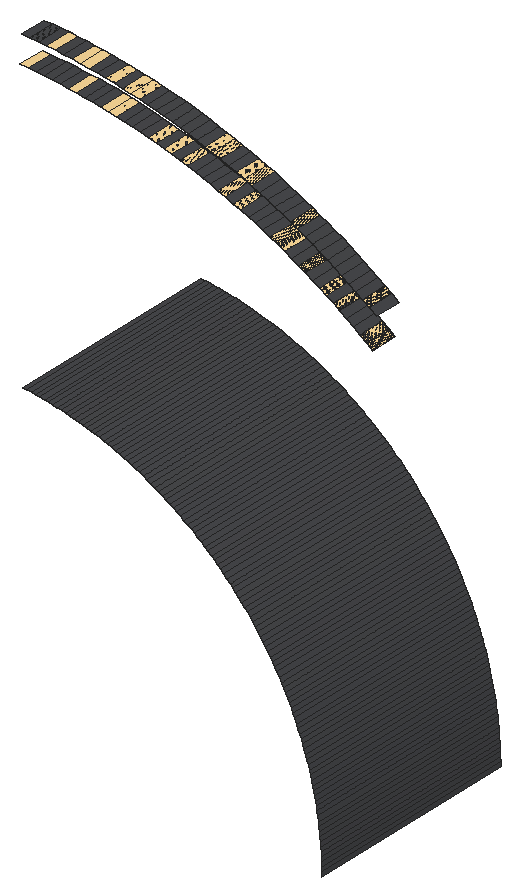
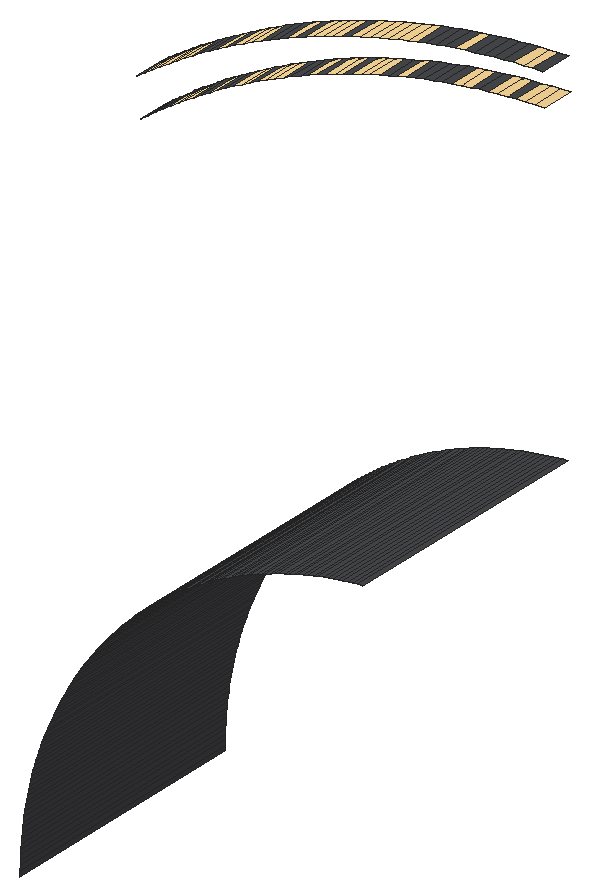
# SketchUp Ruby script. Lengths in inches.
U = 1.inch
M = Sketchup.active_model
def pt(a) = Geom::Point3d.new(a.map { |v| v * U })
def face(e, loops, mat)
  f = e.add_face(loops[0].map { |a| pt(a) })
  loops[1..].each { |l| e.add_face(l.map { |a| pt(a) }).erase! }
  f.material = f.back_material = mat if mat
  f
end
# faces: each face lists its corners as indices into pts; further lists are holes
def faces(e, pts, list, mat = nil) = list.each { |f| face(e, (f[0].is_a?(Array) ? f : [f]).map { |l| l.map { |i| pts[i] } }, mat) }
# xy, xz, yz: faces in a plane at the given z, y or x. An outline is a flat list of corners, or four numbers for a rectangle; further outlines are holes
def ring(l) = l.size == 4 ? [[l[0], l[1]], [l[2], l[1]], [l[2], l[3]], [l[0], l[3]]] : l.each_slice(2).to_a
def flat(e, list, mat, &to3) = list.each { |f| face(e, (f[0].is_a?(Array) ? f : [f]).map { |l| ring(l).map { |u, v| to3.(u, v) } }, mat) }
def xy(e, z, list, mat = nil) = flat(e, list, mat) { |x, y| [x, y, z] }
def xz(e, y, list, mat = nil) = flat(e, list, mat) { |x, z| [x, y, z] }
def yz(e, x, list, mat = nil) = flat(e, list, mat) { |y, z| [x, y, z] }
def lines(e, pts, list) = list.each { |a, b| e.add_line(pt(pts[a]), pt(pts[b])) }
# prism: a flat outline (further loops are holes) pulled along v
def prism(e, loops, v, mat = nil)
  f = face(e, loops, mat); d = Geom::Vector3d.new(v.map { |x| x * U })
  f.pushpull(f.normal.samedirection?(d) ? d.length : -d.length)
end
def box(e, o, s, mat = nil) = prism(e, [[o, [o[0] + s[0], o[1], o[2]], [o[0] + s[0], o[1] + s[1], o[2]], [o[0], o[1] + s[1], o[2]]]], [0, 0, s[2]], mat)
def at(x, y, z, deg = 0) = Geom::Transformation.translation(pt([x, y, z])) * Geom::Transformation.rotation(ORIGIN, Z_AXIS, deg.degrees)
def axes(o, x, y, z) = Geom::Transformation.new([*x, 0, *y, 0, *z, 0, *pt(o).to_a, 1])
def part(name) = M.definitions.add(name)
# library, detail: a bought-in or finely detailed component or shape, given as its bounding box
def library(name, o, s) = part(name).tap { |d| box(d.entities, o, s) }
def detail(e, o, s) = box(e.add_group.entities, o, s)
def put(e, d, t, mat = nil) = e.add_instance(d, t).tap { |i| i.material = mat if mat }
def group(e, t, mat = nil) = e.add_group.tap { |g| g.transformation = t; g.material = mat if mat }.entities
root = M.entities
M.materials.add("1432 AP 8245 TAR ROAD").color = [71, 72, 75]
M.materials.add("Outer Light").color = [251, 217, 152]
yz(root,410.99,[[95.37,411.26,107.37,411.5]],"1432 AP 8245 TAR ROAD")
yz(root,411,[[95.37,410.79,107.37,411.03]],"1432 AP 8245 TAR ROAD")
p = [[410.99,107.37,411.26],[411,107.37,411.03],[411,95.37,411.03],[410.99,95.37,411.26],[410.98,107.37,411.73],[410.99,107.37,411.5],
  [410.99,95.37,411.5],[410.98,95.37,411.73],[410.96,107.37,411.97],[410.96,95.37,411.97],[410.94,107.37,412.2],[410.94,95.37,412.2],
  [410.92,107.37,412.4375],[410.92,95.37,412.4375],[410.9,107.37,412.67],[410.9,95.37,412.67],[410.875,107.37,412.91],[410.875,95.37,412.91],
  [410.85,107.37,413.14],[410.85,95.37,413.14],[410.8125,107.37,413.375],[410.8125,95.37,413.375],[410.78,107.37,413.61],[410.78,95.37,413.61],
  [410.74,107.37,413.84],[410.74,95.37,413.84],[410.7,107.37,414.07],[410.7,95.37,414.07],[410.65,107.37,414.3],[410.65,95.37,414.3],
  [410.61,107.37,414.53],[410.61,95.37,414.53],[410.56,107.37,414.76],[410.56,95.37,414.76],[410.5,107.37,414.99],[410.5,95.37,414.99],
  [410.45,107.37,415.22],[410.45,95.37,415.22],[410.39,107.37,415.45],[410.39,95.37,415.45],[410.32,107.37,415.68],[410.32,95.37,415.68],
  [410.26,107.37,415.9],[410.26,95.37,415.9],[410.19,107.37,416.13],[410.19,95.37,416.13],[410.12,107.37,416.35],[410.12,95.37,416.35],
  [410.04,107.37,416.58],[410.04,95.37,416.58],[409.97,107.37,416.8],[409.97,95.37,416.8],[409.89,107.37,417.02],[409.89,95.37,417.02],
  [409.8,107.37,417.24],[409.8,95.37,417.24],[409.72,107.37,417.46],[409.72,95.37,417.46],[409.63,107.37,417.68],[409.63,95.37,417.68],
  [409.54,107.37,417.9],[409.54,95.37,417.9],[409.44,107.37,418.11],[409.44,95.37,418.11],[409.35,107.37,418.33],[409.35,95.37,418.33],
  [409.25,107.37,418.54],[409.25,95.37,418.54],[409.14,107.37,418.75],[409.14,95.37,418.75],[409.04,107.37,418.96],[409.04,95.37,418.96],
  [408.93,107.37,419.17],[408.93,95.37,419.17],[408.82,107.37,419.38],[408.82,95.37,419.38],[408.7,107.37,419.59],[408.7,95.37,419.59],
  [408.59,107.37,419.79],[408.59,95.37,419.79],[408.47,107.37,420],[408.47,95.37,420],[408.35,107.37,420.2],[408.35,95.37,420.2],
  [408.22,107.37,420.4],[408.22,95.37,420.4],[408.1,107.37,420.6],[408.1,95.37,420.6],[407.97,107.37,420.79],[407.97,95.37,420.79],
  [407.83,107.37,420.99],[407.83,95.37,420.99],[407.7,107.37,421.18],[407.7,95.37,421.18],[407.5625,107.37,421.37],[407.5625,95.37,421.37],
  [407.42,107.37,421.5625],[407.42,95.37,421.5625],[407.28,107.37,421.75],[407.28,95.37,421.75],[407.14,107.37,421.9375],[407.14,95.37,421.9375],
  [406.99,107.37,422.12],[406.99,95.37,422.12],[406.84,107.37,422.3],[406.84,95.37,422.3],[406.6875,107.37,422.48],[406.6875,95.37,422.48],
  [406.53,107.37,422.66],[406.53,95.37,422.66],[406.375,107.37,422.84],[406.375,95.37,422.84],[406.22,107.37,423.01],[406.22,95.37,423.01],
  [406.06,107.37,423.18],[406.06,95.37,423.18],[405.89,107.37,423.35],[405.89,95.37,423.35],[405.73,107.37,423.52],[405.73,95.37,423.52],
  [405.56,107.37,423.69],[405.56,95.37,423.69],[405.39,107.37,423.85],[405.39,95.37,423.85],[405.22,107.37,424.01],[405.22,95.37,424.01],
  [405.04,107.37,424.17],[405.04,95.37,424.17],[404.87,107.37,424.33],[404.87,95.37,424.33],[404.69,107.37,424.48],[404.69,95.37,424.48],
  [404.51,107.37,424.63],[404.51,95.37,424.63],[404.33,107.37,424.78],[404.33,95.37,424.78],[404.14,107.37,424.93],[404.14,95.37,424.93],
  [403.96,107.37,425.07],[403.96,95.37,425.07],[403.77,107.37,425.21],[403.77,95.37,425.21],[403.58,107.37,425.35],[403.58,95.37,425.35],
  [403.39,107.37,425.49],[403.39,95.37,425.49],[403.2,107.37,425.625],[403.2,95.37,425.625],[403,107.37,425.76],[403,95.37,425.76],
  [402.8,107.37,425.89],[402.8,95.37,425.89],[402.61,107.37,426.02],[402.61,95.37,426.02],[402.4,107.37,426.14],[402.4,95.37,426.14],
  [402.2,107.37,426.26],[402.2,95.37,426.26],[402,107.37,426.38],[402,95.37,426.38],[401.8,107.37,426.5],[401.8,95.37,426.5],
  [401.59,107.37,426.61],[401.59,95.37,426.61],[401.38,107.37,426.72],[401.38,95.37,426.72],[401.17,107.37,426.83],[401.17,95.37,426.83],
  [400.96,107.37,426.9375],[400.96,95.37,426.9375],[400.75,107.37,427.04],[400.75,95.37,427.04],[400.54,107.37,427.14],[400.54,95.37,427.14],
  [400.32,107.37,427.24],[400.32,95.37,427.24],[400.11,107.37,427.33],[400.11,95.37,427.33],[399.89,107.37,427.42],[399.89,95.37,427.42],
  [399.67,107.37,427.51],[399.67,95.37,427.51],[399.45,107.37,427.6],[399.45,95.37,427.6],[399.23,107.37,427.68],[399.23,95.37,427.68],
  [399.01,107.37,427.76],[399.01,95.37,427.76],[398.5625,107.37,427.91],[398.79,107.37,427.84],[398.79,95.37,427.84],[398.5625,95.37,427.91],
  [398.34,107.37,427.98],[398.34,95.37,427.98],[398.11,107.37,428.05],[398.11,95.37,428.05],[397.66,107.37,428.18],[397.89,107.37,428.12],
  [397.89,95.37,428.12],[397.66,95.37,428.18],[397.2,107.37,428.29],[397.43,107.37,428.24],[397.43,95.37,428.24],[397.2,95.37,428.29],
  [396.74,107.37,428.4],[396.97,107.37,428.35],[396.97,95.37,428.35],[396.74,95.37,428.4],[396.28,107.37,428.49],[396.51,107.37,428.45],
  [396.51,95.37,428.45],[396.28,95.37,428.49],[395.82,107.37,428.57],[396.05,107.37,428.53],[396.05,95.37,428.53],[395.82,95.37,428.57],
  [395.12,107.37,428.67],[395.35,107.37,428.64],[395.35,95.37,428.64],[395.12,95.37,428.67],[395.58,107.37,428.61],[395.58,95.37,428.61],
  [394.88,107.37,428.69],[394.88,95.37,428.69],[413.39,96.87,437.37],[413.74,96.87,437.1],[413.74,95.37,437.1],[413.39,95.37,437.37],
  [413.39,95.37,437.37],[413.74,95.37,437.1],[413.74,96.87,437.1],[413.39,96.87,437.37],[413.04,96.87,437.63],[413.04,95.37,437.63],
  [413.04,95.37,437.63],[413.04,96.87,437.63],[412.69,96.87,437.89],[412.69,95.37,437.89],[412.69,95.37,437.89],[412.69,96.87,437.89],
  [412.33,96.87,438.15],[412.33,95.37,438.15],[412.33,95.37,438.15],[412.33,96.87,438.15],[411.97,96.87,438.4],[411.97,95.37,438.4],
  [411.97,95.37,438.4],[411.97,96.87,438.4],[411.61,96.87,438.65],[411.61,95.37,438.65],[411.61,95.37,438.65],[411.61,96.87,438.65],
  [411.25,96.87,438.89],[411.25,95.37,438.89],[411.25,95.37,438.89],[411.25,96.87,438.89],[413.94,95.37,438.84],[413.57,95.37,439.11],
  [413.57,96.87,439.11],[413.94,96.87,438.84],[410.875,96.87,439.125],[410.875,95.37,439.125],[410.875,95.37,439.125],[410.875,96.87,439.125],
  [410.5,96.87,439.36],[410.5,95.37,439.36],[410.5,95.37,439.36],[410.5,96.87,439.36],[413.2,95.37,439.375],[413.2,96.87,439.375],
  [413.57,96.87,439.11],[413.2,96.87,439.375],[413.2,95.37,439.375],[413.57,95.37,439.11],[410.13,96.87,439.58],[410.13,95.37,439.58],
  [410.13,95.37,439.58],[410.13,96.87,439.58],[412.82,95.37,439.64],[412.82,96.87,439.64],[412.82,96.87,439.64],[412.82,95.37,439.64],
  [409.75,96.87,439.8],[409.75,95.37,439.8],[409.75,95.37,439.8],[409.75,96.87,439.8],[412.44,95.37,439.89],[412.44,96.87,439.89],
  [412.44,96.87,439.89],[412.44,95.37,439.89],[409.37,96.87,440.02],[409.37,95.37,440.02],[409.37,95.37,440.02],[409.37,96.87,440.02],
  [412.0625,95.37,440.15],[412.0625,96.87,440.15],[412.0625,96.87,440.15],[412.0625,95.37,440.15],[408.98,96.87,440.23],[408.98,95.37,440.23],
  [408.98,95.37,440.23],[408.98,96.87,440.23],[411.68,95.37,440.39],[411.68,96.87,440.39],[411.68,96.87,440.39],[411.68,95.37,440.39],
  [408.6,96.87,440.4375],[408.6,95.37,440.4375],[408.6,95.37,440.4375],[408.6,96.87,440.4375],[408.21,96.87,440.64],[408.21,95.37,440.64],
  [408.21,95.37,440.64],[408.21,96.87,440.64],[411.29,95.37,440.63],[411.29,96.87,440.63],[411.29,96.87,440.63],[411.29,95.37,440.63],
  [407.82,96.87,440.84],[407.82,95.37,440.84],[407.82,95.37,440.84],[407.82,96.87,440.84],[410.9,95.37,440.87],[410.9,96.87,440.87],
  [410.9,96.87,440.87],[410.9,95.37,440.87],[407.42,96.87,441.03],[407.42,95.37,441.03],[407.42,95.37,441.03],[407.42,96.87,441.03],
  [410.5,95.37,441.1],[410.5,96.87,441.1],[410.5,96.87,441.1],[410.5,95.37,441.1],[407.03,96.87,441.21],[407.03,95.37,441.21],
  [407.03,95.37,441.21],[407.03,96.87,441.21],[410.1,95.37,441.33],[410.1,96.87,441.33],[410.1,96.87,441.33],[410.1,95.37,441.33],
  [406.625,96.87,441.4],[406.625,95.37,441.4],[406.625,95.37,441.4],[406.625,96.87,441.4],[409.7,95.37,441.55],[409.7,96.87,441.55],
  [409.7,96.87,441.55],[409.7,95.37,441.55],[406.22,96.87,441.57],[406.22,95.37,441.57],[406.22,95.37,441.57],[406.22,96.87,441.57],
  [405.82,96.87,441.74],[405.82,95.37,441.74],[405.82,95.37,441.74],[405.82,96.87,441.74],[409.3,95.37,441.77],[409.3,96.87,441.77],
  [409.3,96.87,441.77],[409.3,95.37,441.77],[405.41,96.87,441.91],[405.41,95.37,441.91],[405.41,95.37,441.91],[405.41,96.87,441.91],
  [408.89,95.37,441.98],[408.89,96.87,441.98],[408.89,96.87,441.98],[408.89,95.37,441.98],[405.01,96.87,442.07],[405.01,95.37,442.07],
  [405.01,95.37,442.07],[405.01,96.87,442.07],[408.48,95.37,442.18],[408.48,96.87,442.18],[408.48,96.87,442.18],[408.48,95.37,442.18],
  [404.59,96.87,442.22],[404.59,95.37,442.22],[404.59,95.37,442.22],[404.59,96.87,442.22],[404.18,96.87,442.37],[404.18,95.37,442.37],
  [404.18,95.37,442.37],[404.18,96.87,442.37],[408.07,95.37,442.38],[408.07,96.87,442.38],[408.07,96.87,442.38],[408.07,95.37,442.38],
  [403.77,96.87,442.51],[403.77,95.37,442.51],[403.77,95.37,442.51],[403.77,96.87,442.51],[407.65,95.37,442.58],[407.65,96.87,442.58],
  [407.65,96.87,442.58],[407.65,95.37,442.58],[403.35,96.87,442.65],[403.35,95.37,442.65],[403.35,95.37,442.65],[403.35,96.87,442.65],
  [407.24,95.37,442.77],[407.24,96.87,442.77],[407.24,96.87,442.77],[407.24,95.37,442.77],[402.93,96.87,442.79],[402.93,95.37,442.79],
  [402.93,95.37,442.79],[402.93,96.87,442.79],[402.51,96.87,442.91],[402.51,95.37,442.91],[402.51,95.37,442.91],[402.51,96.87,442.91],
  [406.82,95.37,442.95],[406.82,96.87,442.95],[406.82,96.87,442.95],[406.82,95.37,442.95],[402.09,96.87,443.03],[402.09,95.37,443.03],
  [402.09,95.37,443.03],[402.09,96.87,443.03],[406.39,95.37,443.13],[406.39,96.87,443.13],[406.39,96.87,443.13],[406.39,95.37,443.13],
  [401.67,96.87,443.15],[401.67,95.37,443.15],[401.67,95.37,443.15],[401.67,96.87,443.15],[405.97,95.37,443.3],[405.97,96.87,443.3],
  [405.97,96.87,443.3],[405.97,95.37,443.3],[401.25,96.87,443.26],[401.25,95.37,443.26],[401.25,95.37,443.26],[401.25,96.87,443.26],
  [400.82,96.87,443.37],[400.82,95.37,443.37],[400.82,95.37,443.37],[400.82,96.87,443.37],[405.54,95.37,443.47],[405.54,96.87,443.47],
  [405.54,96.87,443.47],[405.54,95.37,443.47],[400.39,96.87,443.47],[400.39,95.37,443.47],[400.39,95.37,443.47],[400.39,96.87,443.47],
  [399.97,96.87,443.56],[399.97,95.37,443.56],[399.97,95.37,443.56],[399.97,96.87,443.56],[405.11,95.37,443.63],[405.11,96.87,443.63],
  [405.11,96.87,443.63],[405.11,95.37,443.63],[399.1,96.87,443.73],[399.54,96.87,443.65],[399.54,95.37,443.65],[399.1,95.37,443.73],
  [399.1,95.37,443.73],[399.54,95.37,443.65],[399.54,96.87,443.65],[399.1,96.87,443.73],[404.68,95.37,443.78],[404.68,96.87,443.78],
  [404.68,96.87,443.78],[404.68,95.37,443.78],[398.67,96.87,443.81],[398.67,95.37,443.81],[398.67,95.37,443.81],[398.67,96.87,443.81],
  [398.24,96.87,443.88],[398.24,95.37,443.88],[398.24,95.37,443.88],[398.24,96.87,443.88],[404.25,95.37,443.93],[404.25,96.87,443.93],
  [404.25,96.87,443.93],[404.25,95.37,443.93],[397.37,96.87,444.01],[397.81,96.87,443.95],[397.81,95.37,443.95],[397.37,95.37,444.01],
  [397.37,95.37,444.01],[397.81,95.37,443.95],[397.81,96.87,443.95],[397.37,96.87,444.01],[403.82,95.37,444.08],[403.82,96.87,444.08],
  [403.82,96.87,444.08],[403.82,95.37,444.08],[396.9375,96.87,444.06],[396.9375,95.37,444.06],[396.9375,95.37,444.06],[396.9375,96.87,444.06],
  [396.07,96.87,444.15],[396.5,96.87,444.11],[396.5,95.37,444.11],[396.07,95.37,444.15],[396.07,95.37,444.15],[396.5,95.37,444.11],
  [396.5,96.87,444.11],[396.07,96.87,444.15],[403.38,95.37,444.22],[403.38,96.87,444.22],[403.38,96.87,444.22],[403.38,95.37,444.22],
  [394.75,96.87,444.25],[395.19,96.87,444.22],[395.19,95.37,444.22],[394.75,95.37,444.25],[395.63,96.87,444.1875],[395.63,95.37,444.1875],
  [395.19,95.37,444.22],[395.63,95.37,444.1875],[395.63,96.87,444.1875],[395.19,96.87,444.22],[402.94,95.37,444.35],[402.94,96.87,444.35],
  [402.94,96.87,444.35],[402.94,95.37,444.35],[402.5,95.37,444.48],[402.5,96.87,444.48],[402.5,96.87,444.48],[402.5,95.37,444.48],
  [402.06,95.37,444.6],[402.06,96.87,444.6],[402.06,96.87,444.6],[402.06,95.37,444.6],[401.62,95.37,444.72],[401.62,96.87,444.72],
  [401.62,96.87,444.72],[401.62,95.37,444.72],[401.17,95.37,444.82],[401.17,96.87,444.82],[401.17,96.87,444.82],[401.17,95.37,444.82],
  [400.72,95.37,444.93],[400.72,96.87,444.93],[400.72,96.87,444.93],[400.72,95.37,444.93],[400.28,95.37,445.03],[400.28,96.87,445.03],
  [400.28,96.87,445.03],[400.28,95.37,445.03],[399.83,95.37,445.12],[399.83,96.87,445.12],[399.83,96.87,445.12],[399.83,95.37,445.12],
  [399.38,95.37,445.21],[399.38,96.87,445.21],[399.38,96.87,445.21],[399.38,95.37,445.21],[398.93,95.37,445.29],[398.93,96.87,445.29],
  [398.93,96.87,445.29],[398.93,95.37,445.29],[398.48,95.37,445.36],[398.48,96.87,445.36],[398.48,96.87,445.36],[398.48,95.37,445.36],
  [398.02,95.37,445.43],[397.57,95.37,445.49],[397.57,96.87,445.49],[398.02,96.87,445.43],[398.02,96.87,445.43],[397.57,96.87,445.49],
  [397.57,95.37,445.49],[398.02,95.37,445.43],[397.11,95.37,445.55],[396.66,95.37,445.6],[396.66,96.87,445.6],[397.11,96.87,445.55],
  [397.11,96.87,445.55],[396.66,96.87,445.6],[396.66,95.37,445.6],[397.11,95.37,445.55],[396.2,95.37,445.65],[395.75,95.37,445.68],
  [395.75,96.87,445.68],[396.2,96.87,445.65],[396.2,96.87,445.65],[395.75,96.87,445.68],[395.75,95.37,445.68],[396.2,95.37,445.65],
  [395.29,95.37,445.72],[394.83,95.37,445.74],[394.83,96.87,445.74],[395.29,96.87,445.72],[395.29,96.87,445.72],[394.83,96.87,445.74],
  [394.83,95.37,445.74],[395.29,95.37,445.72]]
faces(root,p,[[0,1,2,3],[4,5,6,7],[8,4,7,9],[10,8,9,11],[12,10,11,13],[14,12,13,15],[16,14,15,17],[18,16,17,19],
  [20,18,19,21],[22,20,21,23],[24,22,23,25],[26,24,25,27],[28,26,27,29],[30,28,29,31],[32,30,31,33],[34,32,33,35],
  [36,34,35,37],[38,36,37,39],[40,38,39,41],[42,40,41,43],[44,42,43,45],[46,44,45,47],[48,46,47,49],[50,48,49,51],
  [52,50,51,53],[54,52,53,55],[56,54,55,57],[58,56,57,59],[60,58,59,61],[62,60,61,63],[64,62,63,65],[66,64,65,67],
  [68,66,67,69],[70,68,69,71],[72,70,71,73],[74,72,73,75],[76,74,75,77],[78,76,77,79],[80,78,79,81],[82,80,81,83],
  [84,82,83,85],[86,84,85,87],[88,86,87,89],[90,88,89,91],[92,90,91,93],[94,92,93,95],[96,94,95,97],[98,96,97,99],
  [100,98,99,101],[102,100,101,103],[104,102,103,105],[106,104,105,107],[108,106,107,109],[110,108,109,111],[112,110,111,113],[114,112,113,115],
  [116,114,115,117],[118,116,117,119],[120,118,119,121],[122,120,121,123],[124,122,123,125],[126,124,125,127],[128,126,127,129],[130,128,129,131],
  [132,130,131,133],[134,132,133,135],[136,134,135,137],[138,136,137,139],[140,138,139,141],[142,140,141,143],[144,142,143,145],[146,144,145,147],
  [148,146,147,149],[150,148,149,151],[152,150,151,153],[154,152,153,155],[156,154,155,157],[158,156,157,159],[160,158,159,161],[162,160,161,163],
  [164,162,163,165],[166,164,165,167],[168,166,167,169],[170,168,169,171],[172,170,171,173],[174,172,173,175],[176,174,175,177],[178,176,177,179],
  [180,178,179,181],[182,180,181,183],[184,182,183,185],[186,184,185,187],[188,189,190,191],[189,186,187,190],[192,188,191,193],[194,192,193,195],
  [196,197,198,199],[197,194,195,198],[200,201,202,203],[201,196,199,202],[204,205,206,207],[205,200,203,206],[208,209,210,211],[209,204,207,210],
  [212,213,214,215],[213,208,211,214],[216,217,218,219],[217,220,221,218],[220,212,215,221],[222,216,219,223],[228,229,230,231],[234,228,231,235],
  [238,234,235,239],[242,238,239,243],[246,242,243,247],[250,246,247,251],[254,250,251,255],[256,257,258,259],[262,254,255,263],[266,262,263,267],
  [257,268,269,258],[276,266,267,277],[268,278,279,269],[284,276,277,285],[278,286,287,279],[292,284,285,293],[286,294,295,287],[300,292,293,301],
  [294,302,303,295],[308,300,301,309],[312,308,309,313],[302,314,315,303],[320,312,313,321],[314,322,323,315],[328,320,321,329],[322,330,331,323],
  [336,328,329,337],[330,338,339,331],[344,336,337,345],[338,346,347,339],[352,344,345,353],[356,352,353,357],[346,358,359,347],[364,356,357,365],
  [358,366,367,359],[372,364,365,373],[366,374,375,367],[380,372,373,381],[384,380,381,385],[374,386,387,375],[392,384,385,393],[386,394,395,387],
  [400,392,393,401],[394,402,403,395],[408,400,401,409],[412,408,409,413],[402,414,415,403],[420,412,413,421],[414,422,423,415],[428,420,421,429],
  [422,430,431,423],[436,428,429,437],[440,436,437,441],[430,442,443,431],[448,440,441,449],[452,448,449,453],[442,454,455,443],[462,463,464,465],
  [463,452,453,464],[454,466,467,455],[472,462,465,473],[476,472,473,477],[466,478,479,467],[486,487,488,489],[487,476,477,488],[478,490,491,479],
  [496,486,489,497],[502,503,504,505],[503,496,497,504],[490,506,507,491],[516,517,518,519],[517,502,505,518],[506,520,521,507],[520,524,525,521],
  [524,528,529,525],[528,532,533,529],[532,536,537,533],[536,540,541,537],[540,544,545,541],[544,548,549,545],[548,552,553,549],[552,556,557,553],
  [556,560,561,557],[564,565,566,567],[560,564,567,561],[572,573,574,575],[565,572,575,566],[580,581,582,583],[573,580,583,574],[588,589,590,591],
  [581,588,591,582]],"1432 AP 8245 TAR ROAD")
faces(root,p,[[224,225,226,227],[232,224,227,233],[236,232,233,237],[240,236,237,241],[244,240,241,245],[248,244,245,249],[252,248,249,253],[260,252,253,261],
  [264,260,261,265],[270,271,272,273],[274,264,265,275],[271,280,281,272],[282,274,275,283],[280,288,289,281],[290,282,283,291],[288,296,297,289],
  [298,290,291,299],[296,304,305,297],[306,298,299,307],[310,306,307,311],[304,316,317,305],[318,310,311,319],[316,324,325,317],[326,318,319,327],
  [324,332,333,325],[334,326,327,335],[332,340,341,333],[342,334,335,343],[340,348,349,341],[350,342,343,351],[354,350,351,355],[348,360,361,349],
  [362,354,355,363],[360,368,369,361],[370,362,363,371],[368,376,377,369],[378,370,371,379],[382,378,379,383],[376,388,389,377],[390,382,383,391],
  [388,396,397,389],[398,390,391,399],[396,404,405,397],[406,398,399,407],[410,406,407,411],[404,416,417,405],[418,410,411,419],[416,424,425,417],
  [426,418,419,427],[424,432,433,425],[434,426,427,435],[438,434,435,439],[432,444,445,433],[446,438,439,447],[450,446,447,451],[444,456,457,445],
  [458,459,460,461],[459,450,451,460],[456,468,469,457],[470,458,461,471],[474,470,471,475],[468,480,481,469],[482,483,484,485],[483,474,475,484],
  [480,492,493,481],[494,482,485,495],[498,499,500,501],[499,494,495,500],[492,508,509,493],[510,511,512,513],[511,514,515,512],[514,498,501,515],
  [508,522,523,509],[522,526,527,523],[526,530,531,527],[530,534,535,531],[534,538,539,535],[538,542,543,539],[542,546,547,543],[546,550,551,547],
  [550,554,555,551],[554,558,559,555],[558,562,563,559],[568,569,570,571],[562,568,571,563],[576,577,578,579],[569,576,579,570],[584,585,586,587],
  [577,584,587,578],[592,593,594,595],[585,592,595,586]],"Outer Light")
